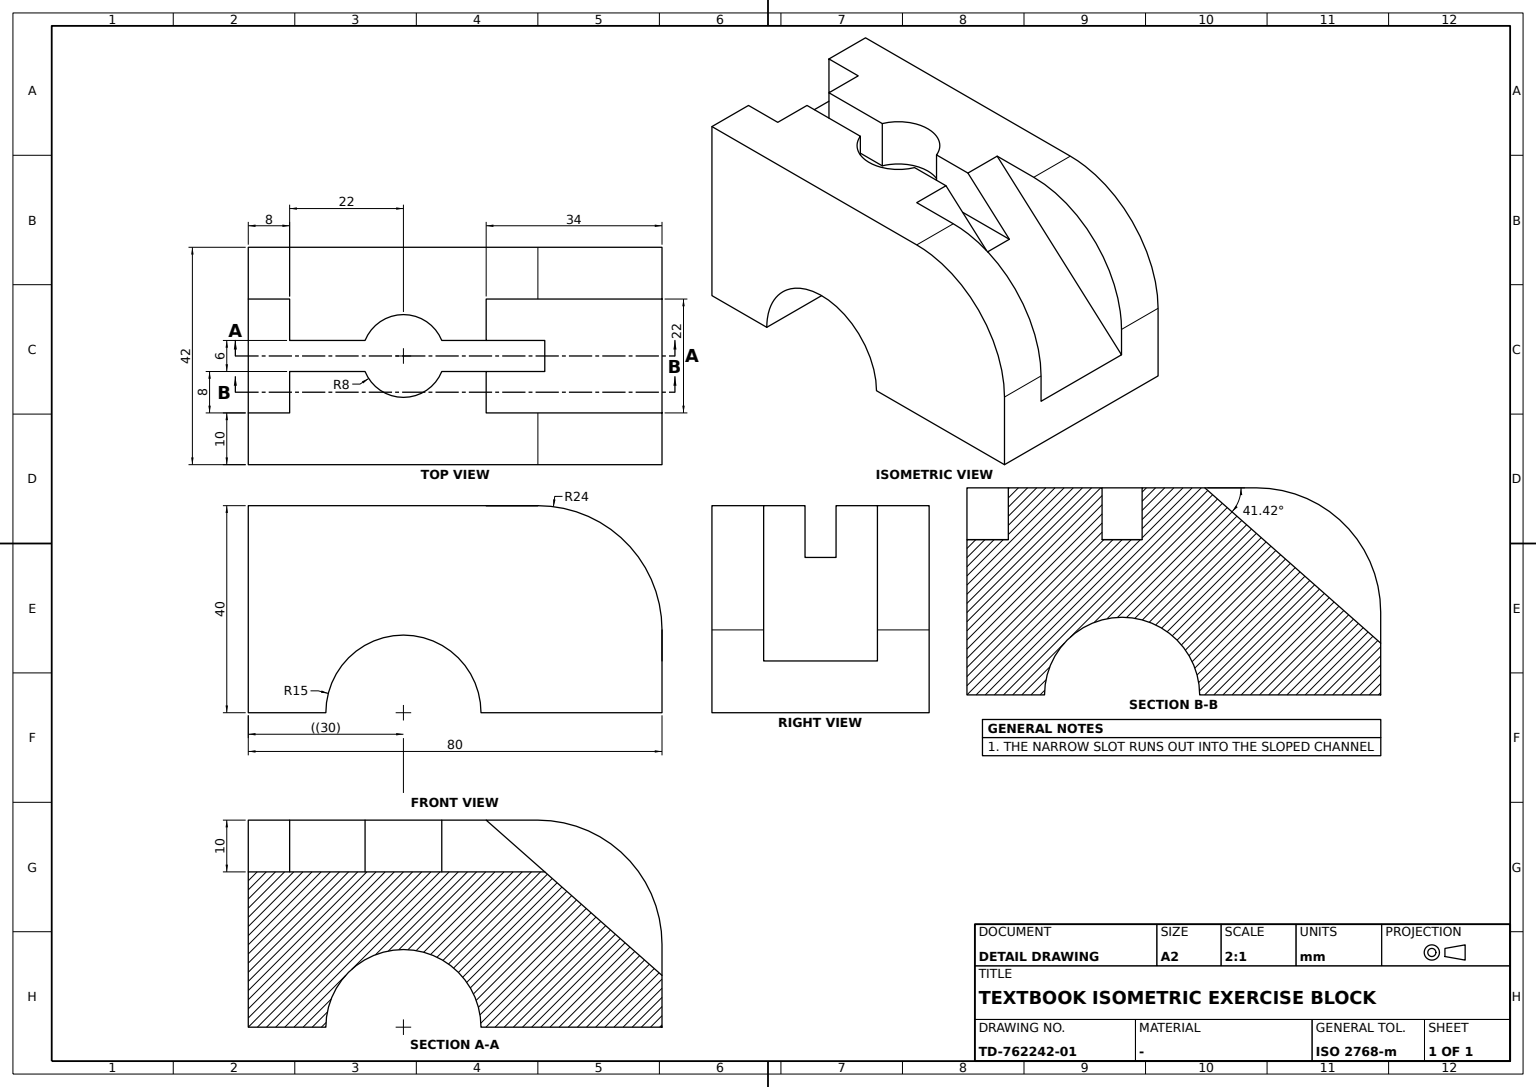
ISO-10303-21;
HEADER;
FILE_DESCRIPTION((''),'2;1');
FILE_NAME('','',(''),(''),'','','');
FILE_SCHEMA(('AUTOMOTIVE_DESIGN'));
ENDSEC;
DATA;
#1=APPLICATION_CONTEXT('');
#2=PRODUCT_CONTEXT('',#1,'mechanical');
#3=PRODUCT('','','',(#2));
#4=PRODUCT_DEFINITION_FORMATION('','',#3);
#5=PRODUCT_DEFINITION_CONTEXT('',#1,'design');
#6=PRODUCT_DEFINITION('','',#4,#5);
#7=PRODUCT_DEFINITION_SHAPE('','',#6);
#8=(LENGTH_UNIT()NAMED_UNIT(*)SI_UNIT(.MILLI.,.METRE.));
#9=(NAMED_UNIT(*)PLANE_ANGLE_UNIT()SI_UNIT($,.RADIAN.));
#10=(NAMED_UNIT(*)SI_UNIT($,.STERADIAN.)SOLID_ANGLE_UNIT());
#11=UNCERTAINTY_MEASURE_WITH_UNIT(LENGTH_MEASURE(0.005),#8,'distance_accuracy_value','');
#12=(GEOMETRIC_REPRESENTATION_CONTEXT(3)GLOBAL_UNCERTAINTY_ASSIGNED_CONTEXT((#11))GLOBAL_UNIT_ASSIGNED_CONTEXT((#8,#9,#10))REPRESENTATION_CONTEXT('',''));
#13=CARTESIAN_POINT('',(21.,0.,0.));
#14=VERTEX_POINT('',#13);
#15=CARTESIAN_POINT('',(21.,15.,0.));
#16=VERTEX_POINT('',#15);
#17=DIRECTION('',(0.,1.,0.));
#18=VECTOR('',#17,1000.);
#19=LINE('',#13,#18);
#20=EDGE_CURVE('',#14,#16,#19,.T.);
#21=ORIENTED_EDGE('',*,*,#20,.T.);
#22=CARTESIAN_POINT('',(21.,45.,0.));
#23=VERTEX_POINT('',#22);
#24=CARTESIAN_POINT('',(21.,30.,0.));
#25=DIRECTION('',(1.,0.,0.));
#26=DIRECTION('',(0.,0.,-1.));
#27=AXIS2_PLACEMENT_3D('',#24,#25,#26);
#28=CIRCLE('',#27,15.);
#29=EDGE_CURVE('',#23,#16,#28,.T.);
#30=ORIENTED_EDGE('',*,*,#29,.F.);
#31=CARTESIAN_POINT('',(21.,80.,0.));
#32=VERTEX_POINT('',#31);
#33=EDGE_CURVE('',#23,#32,#19,.T.);
#34=ORIENTED_EDGE('',*,*,#33,.T.);
#35=CARTESIAN_POINT('',(21.,80.,16.));
#36=VERTEX_POINT('',#35);
#37=DIRECTION('',(0.,0.,1.));
#38=VECTOR('',#37,1000.);
#39=LINE('',#31,#38);
#40=EDGE_CURVE('',#32,#36,#39,.T.);
#41=ORIENTED_EDGE('',*,*,#40,.T.);
#42=CARTESIAN_POINT('',(21.,56.,40.));
#43=VERTEX_POINT('',#42);
#44=CARTESIAN_POINT('',(21.,56.,16.));
#45=AXIS2_PLACEMENT_3D('',#44,#25,#26);
#46=CIRCLE('',#45,24.);
#47=EDGE_CURVE('',#36,#43,#46,.T.);
#48=ORIENTED_EDGE('',*,*,#47,.T.);
#49=CARTESIAN_POINT('',(21.,0.,40.));
#50=VERTEX_POINT('',#49);
#51=DIRECTION('',(0.,-1.,0.));
#52=VECTOR('',#51,1000.);
#53=LINE('',#49,#52);
#54=EDGE_CURVE('',#43,#50,#53,.T.);
#55=ORIENTED_EDGE('',*,*,#54,.T.);
#56=VECTOR('',#26,1000.);
#57=LINE('',#13,#56);
#58=EDGE_CURVE('',#50,#14,#57,.T.);
#59=ORIENTED_EDGE('',*,*,#58,.T.);
#60=EDGE_LOOP('',(#21,#30,#34,#41,#48,#55,#59));
#61=FACE_BOUND('',#60,.T.);
#62=AXIS2_PLACEMENT_3D('',#13,#25,#17);
#63=PLANE('',#62);
#64=ADVANCED_FACE('',(#61),#63,.T.);
#65=CARTESIAN_POINT('',(3.,22.583802,40.));
#66=VERTEX_POINT('',#65);
#67=CARTESIAN_POINT('',(3.,37.416198,40.));
#68=VERTEX_POINT('',#67);
#69=CARTESIAN_POINT('',(0.,30.,40.));
#70=AXIS2_PLACEMENT_3D('',#69,#37,#25);
#71=CIRCLE('',#70,8.);
#72=EDGE_CURVE('',#66,#68,#71,.T.);
#73=ORIENTED_EDGE('',*,*,#72,.T.);
#74=CARTESIAN_POINT('',(3.,37.416198,30.));
#75=VERTEX_POINT('',#74);
#76=LINE('',#67,#38);
#77=EDGE_CURVE('',#68,#75,#76,.F.);
#78=ORIENTED_EDGE('',*,*,#77,.T.);
#79=CARTESIAN_POINT('',(3.,22.583802,30.));
#80=VERTEX_POINT('',#79);
#81=CARTESIAN_POINT('',(0.,30.,30.));
#82=AXIS2_PLACEMENT_3D('',#81,#37,#25);
#83=CIRCLE('',#82,8.);
#84=EDGE_CURVE('',#80,#75,#83,.T.);
#85=ORIENTED_EDGE('',*,*,#84,.F.);
#86=LINE('',#65,#38);
#87=EDGE_CURVE('',#66,#80,#86,.F.);
#88=ORIENTED_EDGE('',*,*,#87,.F.);
#89=EDGE_LOOP('',(#73,#78,#85,#88));
#90=FACE_BOUND('',#89,.T.);
#91=CARTESIAN_POINT('',(0.,30.,35.));
#92=AXIS2_PLACEMENT_3D('',#91,#37,#25);
#93=CYLINDRICAL_SURFACE('',#92,8.);
#94=ADVANCED_FACE('',(#90),#93,.F.);
#95=CARTESIAN_POINT('',(-11.,56.,40.));
#96=VERTEX_POINT('',#95);
#97=CARTESIAN_POINT('',(-11.,80.,16.));
#98=VERTEX_POINT('',#97);
#99=CARTESIAN_POINT('',(-11.,56.,16.));
#100=DIRECTION('',(-1.,0.,0.));
#101=AXIS2_PLACEMENT_3D('',#99,#100,#37);
#102=CIRCLE('',#101,24.);
#103=EDGE_CURVE('',#96,#98,#102,.T.);
#104=ORIENTED_EDGE('',*,*,#103,.T.);
#105=CARTESIAN_POINT('',(-21.,80.,16.));
#106=VERTEX_POINT('',#105);
#107=CARTESIAN_POINT('',(0.,80.,16.));
#108=VECTOR('',#25,1000.);
#109=LINE('',#107,#108);
#110=EDGE_CURVE('',#106,#98,#109,.T.);
#111=ORIENTED_EDGE('',*,*,#110,.F.);
#112=CARTESIAN_POINT('',(-21.,56.,40.));
#113=VERTEX_POINT('',#112);
#114=CARTESIAN_POINT('',(-21.,56.,16.));
#115=AXIS2_PLACEMENT_3D('',#114,#25,#26);
#116=CIRCLE('',#115,24.);
#117=EDGE_CURVE('',#106,#113,#116,.T.);
#118=ORIENTED_EDGE('',*,*,#117,.T.);
#119=CARTESIAN_POINT('',(0.,56.,40.));
#120=LINE('',#119,#108);
#121=EDGE_CURVE('',#113,#96,#120,.T.);
#122=ORIENTED_EDGE('',*,*,#121,.T.);
#123=EDGE_LOOP('',(#104,#111,#118,#122));
#124=FACE_BOUND('',#123,.T.);
#125=CARTESIAN_POINT('',(0.,56.,16.));
#126=AXIS2_PLACEMENT_3D('',#125,#25,#37);
#127=CYLINDRICAL_SURFACE('',#126,24.);
#128=ADVANCED_FACE('',(#124),#127,.T.);
#129=CARTESIAN_POINT('',(-3.,46.,40.));
#130=VERTEX_POINT('',#129);
#131=CARTESIAN_POINT('',(-3.,57.333333,30.));
#132=VERTEX_POINT('',#131);
#133=DIRECTION('',(0.,0.749837855,-0.661621637));
#134=VECTOR('',#133,1000.);
#135=LINE('',#129,#134);
#136=EDGE_CURVE('',#130,#132,#135,.T.);
#137=ORIENTED_EDGE('',*,*,#136,.F.);
#138=CARTESIAN_POINT('',(-3.,37.416198,40.));
#139=VERTEX_POINT('',#138);
#140=CARTESIAN_POINT('',(-3.,57.416198,40.));
#141=LINE('',#140,#52);
#142=EDGE_CURVE('',#130,#139,#141,.T.);
#143=ORIENTED_EDGE('',*,*,#142,.T.);
#144=CARTESIAN_POINT('',(-3.,37.416198,30.));
#145=VERTEX_POINT('',#144);
#146=LINE('',#138,#38);
#147=EDGE_CURVE('',#139,#145,#146,.F.);
#148=ORIENTED_EDGE('',*,*,#147,.T.);
#149=CARTESIAN_POINT('',(-3.,57.416198,30.));
#150=LINE('',#149,#52);
#151=EDGE_CURVE('',#132,#145,#150,.T.);
#152=ORIENTED_EDGE('',*,*,#151,.F.);
#153=EDGE_LOOP('',(#137,#143,#148,#152));
#154=FACE_BOUND('',#153,.T.);
#155=AXIS2_PLACEMENT_3D('',#140,#25,#51);
#156=PLANE('',#155);
#157=ADVANCED_FACE('',(#154),#156,.T.);
#158=ORIENTED_EDGE('',*,*,#84,.T.);
#159=CARTESIAN_POINT('',(3.,57.333333,30.));
#160=VERTEX_POINT('',#159);
#161=CARTESIAN_POINT('',(3.,8.,30.));
#162=LINE('',#161,#18);
#163=EDGE_CURVE('',#75,#160,#162,.T.);
#164=ORIENTED_EDGE('',*,*,#163,.T.);
#165=CARTESIAN_POINT('',(21.,57.333333,30.));
#166=LINE('',#165,#108);
#167=EDGE_CURVE('',#132,#160,#166,.T.);
#168=ORIENTED_EDGE('',*,*,#167,.F.);
#169=ORIENTED_EDGE('',*,*,#151,.T.);
#170=CARTESIAN_POINT('',(-3.,22.583802,30.));
#171=VERTEX_POINT('',#170);
#172=EDGE_CURVE('',#145,#171,#83,.T.);
#173=ORIENTED_EDGE('',*,*,#172,.T.);
#174=CARTESIAN_POINT('',(-3.,8.,30.));
#175=VERTEX_POINT('',#174);
#176=EDGE_CURVE('',#171,#175,#150,.T.);
#177=ORIENTED_EDGE('',*,*,#176,.T.);
#178=CARTESIAN_POINT('',(-11.,8.,30.));
#179=VERTEX_POINT('',#178);
#180=LINE('',#161,#108);
#181=EDGE_CURVE('',#179,#175,#180,.T.);
#182=ORIENTED_EDGE('',*,*,#181,.F.);
#183=CARTESIAN_POINT('',(-11.,0.,30.));
#184=VERTEX_POINT('',#183);
#185=LINE('',#183,#52);
#186=EDGE_CURVE('',#179,#184,#185,.T.);
#187=ORIENTED_EDGE('',*,*,#186,.T.);
#188=CARTESIAN_POINT('',(11.,0.,30.));
#189=VERTEX_POINT('',#188);
#190=CARTESIAN_POINT('',(0.,0.,30.));
#191=VECTOR('',#100,1000.);
#192=LINE('',#190,#191);
#193=EDGE_CURVE('',#189,#184,#192,.T.);
#194=ORIENTED_EDGE('',*,*,#193,.F.);
#195=CARTESIAN_POINT('',(11.,8.,30.));
#196=VERTEX_POINT('',#195);
#197=LINE('',#188,#18);
#198=EDGE_CURVE('',#189,#196,#197,.T.);
#199=ORIENTED_EDGE('',*,*,#198,.T.);
#200=VERTEX_POINT('',#161);
#201=EDGE_CURVE('',#200,#196,#180,.T.);
#202=ORIENTED_EDGE('',*,*,#201,.F.);
#203=EDGE_CURVE('',#200,#80,#162,.T.);
#204=ORIENTED_EDGE('',*,*,#203,.T.);
#205=EDGE_LOOP('',(#158,#164,#168,#169,#173,#177,#182,#187,#194,#199,#202,#204));
#206=FACE_BOUND('',#205,.T.);
#207=AXIS2_PLACEMENT_3D('',#190,#37,#25);
#208=PLANE('',#207);
#209=ADVANCED_FACE('',(#206),#208,.T.);
#210=ORIENTED_EDGE('',*,*,#186,.F.);
#211=CARTESIAN_POINT('',(-11.,8.,40.));
#212=VERTEX_POINT('',#211);
#213=CARTESIAN_POINT('',(-11.,8.,0.));
#214=LINE('',#213,#56);
#215=EDGE_CURVE('',#212,#179,#214,.T.);
#216=ORIENTED_EDGE('',*,*,#215,.F.);
#217=CARTESIAN_POINT('',(-11.,0.,40.));
#218=VERTEX_POINT('',#217);
#219=CARTESIAN_POINT('',(-11.,80.,40.));
#220=LINE('',#219,#52);
#221=EDGE_CURVE('',#212,#218,#220,.T.);
#222=ORIENTED_EDGE('',*,*,#221,.T.);
#223=LINE('',#217,#56);
#224=EDGE_CURVE('',#218,#184,#223,.T.);
#225=ORIENTED_EDGE('',*,*,#224,.T.);
#226=EDGE_LOOP('',(#210,#216,#222,#225));
#227=FACE_BOUND('',#226,.T.);
#228=CARTESIAN_POINT('',(-11.,0.,0.));
#229=AXIS2_PLACEMENT_3D('',#228,#100,#51);
#230=PLANE('',#229);
#231=ADVANCED_FACE('',(#227),#230,.F.);
#232=CARTESIAN_POINT('',(-21.,0.,0.));
#233=VERTEX_POINT('',#232);
#234=CARTESIAN_POINT('',(0.,0.,0.));
#235=LINE('',#234,#108);
#236=EDGE_CURVE('',#233,#14,#235,.T.);
#237=ORIENTED_EDGE('',*,*,#236,.F.);
#238=CARTESIAN_POINT('',(-21.,15.,0.));
#239=VERTEX_POINT('',#238);
#240=LINE('',#232,#18);
#241=EDGE_CURVE('',#233,#239,#240,.T.);
#242=ORIENTED_EDGE('',*,*,#241,.T.);
#243=LINE('',#238,#108);
#244=EDGE_CURVE('',#239,#16,#243,.T.);
#245=ORIENTED_EDGE('',*,*,#244,.T.);
#246=ORIENTED_EDGE('',*,*,#20,.F.);
#247=EDGE_LOOP('',(#237,#242,#245,#246));
#248=FACE_BOUND('',#247,.T.);
#249=AXIS2_PLACEMENT_3D('',#234,#26,#17);
#250=PLANE('',#249);
#251=ADVANCED_FACE('',(#248),#250,.T.);
#252=ORIENTED_EDGE('',*,*,#201,.T.);
#253=CARTESIAN_POINT('',(11.,8.,40.));
#254=VERTEX_POINT('',#253);
#255=LINE('',#253,#56);
#256=EDGE_CURVE('',#254,#196,#255,.T.);
#257=ORIENTED_EDGE('',*,*,#256,.F.);
#258=CARTESIAN_POINT('',(3.,8.,40.));
#259=VERTEX_POINT('',#258);
#260=LINE('',#258,#108);
#261=EDGE_CURVE('',#259,#254,#260,.T.);
#262=ORIENTED_EDGE('',*,*,#261,.F.);
#263=LINE('',#258,#56);
#264=EDGE_CURVE('',#259,#200,#263,.T.);
#265=ORIENTED_EDGE('',*,*,#264,.T.);
#266=EDGE_LOOP('',(#252,#257,#262,#265));
#267=FACE_BOUND('',#266,.T.);
#268=AXIS2_PLACEMENT_3D('',#258,#17,#25);
#269=PLANE('',#268);
#270=ADVANCED_FACE('',(#267),#269,.F.);
#271=CARTESIAN_POINT('',(11.,80.,16.));
#272=VERTEX_POINT('',#271);
#273=EDGE_CURVE('',#36,#272,#109,.F.);
#274=ORIENTED_EDGE('',*,*,#273,.F.);
#275=ORIENTED_EDGE('',*,*,#40,.F.);
#276=CARTESIAN_POINT('',(-21.,80.,0.));
#277=VERTEX_POINT('',#276);
#278=CARTESIAN_POINT('',(0.,80.,0.));
#279=LINE('',#278,#108);
#280=EDGE_CURVE('',#277,#32,#279,.T.);
#281=ORIENTED_EDGE('',*,*,#280,.F.);
#282=LINE('',#276,#38);
#283=EDGE_CURVE('',#277,#106,#282,.T.);
#284=ORIENTED_EDGE('',*,*,#283,.T.);
#285=ORIENTED_EDGE('',*,*,#110,.T.);
#286=CARTESIAN_POINT('',(-11.,80.,10.));
#287=VERTEX_POINT('',#286);
#288=CARTESIAN_POINT('',(-11.,80.,0.));
#289=LINE('',#288,#38);
#290=EDGE_CURVE('',#287,#98,#289,.T.);
#291=ORIENTED_EDGE('',*,*,#290,.F.);
#292=CARTESIAN_POINT('',(11.,80.,10.));
#293=VERTEX_POINT('',#292);
#294=CARTESIAN_POINT('',(21.,80.,10.));
#295=LINE('',#294,#191);
#296=EDGE_CURVE('',#293,#287,#295,.T.);
#297=ORIENTED_EDGE('',*,*,#296,.F.);
#298=CARTESIAN_POINT('',(11.,80.,0.));
#299=LINE('',#298,#38);
#300=EDGE_CURVE('',#293,#272,#299,.T.);
#301=ORIENTED_EDGE('',*,*,#300,.T.);
#302=EDGE_LOOP('',(#274,#275,#281,#284,#285,#291,#297,#301));
#303=FACE_BOUND('',#302,.T.);
#304=AXIS2_PLACEMENT_3D('',#278,#17,#37);
#305=PLANE('',#304);
#306=ADVANCED_FACE('',(#303),#305,.T.);
#307=CARTESIAN_POINT('',(-21.,0.,40.));
#308=VERTEX_POINT('',#307);
#309=LINE('',#232,#56);
#310=EDGE_CURVE('',#308,#233,#309,.T.);
#311=ORIENTED_EDGE('',*,*,#310,.T.);
#312=ORIENTED_EDGE('',*,*,#236,.T.);
#313=ORIENTED_EDGE('',*,*,#58,.F.);
#314=CARTESIAN_POINT('',(11.,0.,40.));
#315=VERTEX_POINT('',#314);
#316=CARTESIAN_POINT('',(0.,0.,40.));
#317=LINE('',#316,#108);
#318=EDGE_CURVE('',#315,#50,#317,.T.);
#319=ORIENTED_EDGE('',*,*,#318,.F.);
#320=CARTESIAN_POINT('',(11.,0.,0.));
#321=LINE('',#320,#56);
#322=EDGE_CURVE('',#315,#189,#321,.T.);
#323=ORIENTED_EDGE('',*,*,#322,.T.);
#324=ORIENTED_EDGE('',*,*,#193,.T.);
#325=ORIENTED_EDGE('',*,*,#224,.F.);
#326=EDGE_CURVE('',#308,#218,#317,.T.);
#327=ORIENTED_EDGE('',*,*,#326,.F.);
#328=EDGE_LOOP('',(#311,#312,#313,#319,#323,#324,#325,#327));
#329=FACE_BOUND('',#328,.T.);
#330=AXIS2_PLACEMENT_3D('',#316,#51,#26);
#331=PLANE('',#330);
#332=ADVANCED_FACE('',(#329),#331,.T.);
#333=ORIENTED_EDGE('',*,*,#87,.T.);
#334=ORIENTED_EDGE('',*,*,#203,.F.);
#335=ORIENTED_EDGE('',*,*,#264,.F.);
#336=LINE('',#258,#18);
#337=EDGE_CURVE('',#259,#66,#336,.T.);
#338=ORIENTED_EDGE('',*,*,#337,.T.);
#339=EDGE_LOOP('',(#333,#334,#335,#338));
#340=FACE_BOUND('',#339,.T.);
#341=AXIS2_PLACEMENT_3D('',#258,#100,#17);
#342=PLANE('',#341);
#343=ADVANCED_FACE('',(#340),#342,.T.);
#344=CARTESIAN_POINT('',(11.,46.,40.));
#345=VERTEX_POINT('',#344);
#346=LINE('',#344,#134);
#347=EDGE_CURVE('',#345,#293,#346,.T.);
#348=ORIENTED_EDGE('',*,*,#347,.F.);
#349=CARTESIAN_POINT('',(11.,56.,40.));
#350=VERTEX_POINT('',#349);
#351=LINE('',#314,#52);
#352=EDGE_CURVE('',#350,#345,#351,.T.);
#353=ORIENTED_EDGE('',*,*,#352,.F.);
#354=CARTESIAN_POINT('',(11.,56.,16.));
#355=AXIS2_PLACEMENT_3D('',#354,#25,#26);
#356=CIRCLE('',#355,24.);
#357=EDGE_CURVE('',#272,#350,#356,.T.);
#358=ORIENTED_EDGE('',*,*,#357,.F.);
#359=ORIENTED_EDGE('',*,*,#300,.F.);
#360=EDGE_LOOP('',(#348,#353,#358,#359));
#361=FACE_BOUND('',#360,.T.);
#362=AXIS2_PLACEMENT_3D('',#320,#25,#17);
#363=PLANE('',#362);
#364=ADVANCED_FACE('',(#361),#363,.F.);
#365=ORIENTED_EDGE('',*,*,#326,.T.);
#366=ORIENTED_EDGE('',*,*,#221,.F.);
#367=CARTESIAN_POINT('',(-3.,8.,40.));
#368=VERTEX_POINT('',#367);
#369=EDGE_CURVE('',#212,#368,#260,.T.);
#370=ORIENTED_EDGE('',*,*,#369,.T.);
#371=CARTESIAN_POINT('',(-3.,22.583802,40.));
#372=VERTEX_POINT('',#371);
#373=EDGE_CURVE('',#372,#368,#141,.T.);
#374=ORIENTED_EDGE('',*,*,#373,.F.);
#375=EDGE_CURVE('',#139,#372,#71,.T.);
#376=ORIENTED_EDGE('',*,*,#375,.F.);
#377=ORIENTED_EDGE('',*,*,#142,.F.);
#378=CARTESIAN_POINT('',(-11.,46.,40.));
#379=VERTEX_POINT('',#378);
#380=CARTESIAN_POINT('',(0.,46.,40.));
#381=LINE('',#380,#191);
#382=EDGE_CURVE('',#130,#379,#381,.T.);
#383=ORIENTED_EDGE('',*,*,#382,.T.);
#384=EDGE_CURVE('',#96,#379,#220,.T.);
#385=ORIENTED_EDGE('',*,*,#384,.F.);
#386=ORIENTED_EDGE('',*,*,#121,.F.);
#387=LINE('',#307,#52);
#388=EDGE_CURVE('',#113,#308,#387,.T.);
#389=ORIENTED_EDGE('',*,*,#388,.T.);
#390=EDGE_LOOP('',(#365,#366,#370,#374,#376,#377,#383,#385,#386,#389));
#391=FACE_BOUND('',#390,.T.);
#392=CARTESIAN_POINT('',(0.,80.,40.));
#393=AXIS2_PLACEMENT_3D('',#392,#37,#51);
#394=PLANE('',#393);
#395=ADVANCED_FACE('',(#391),#394,.T.);
#396=ORIENTED_EDGE('',*,*,#33,.F.);
#397=CARTESIAN_POINT('',(-21.,45.,0.));
#398=VERTEX_POINT('',#397);
#399=LINE('',#397,#108);
#400=EDGE_CURVE('',#23,#398,#399,.F.);
#401=ORIENTED_EDGE('',*,*,#400,.T.);
#402=EDGE_CURVE('',#398,#277,#240,.T.);
#403=ORIENTED_EDGE('',*,*,#402,.T.);
#404=ORIENTED_EDGE('',*,*,#280,.T.);
#405=EDGE_LOOP('',(#396,#401,#403,#404));
#406=FACE_BOUND('',#405,.T.);
#407=ADVANCED_FACE('',(#406),#250,.T.);
#408=LINE('',#371,#38);
#409=EDGE_CURVE('',#372,#171,#408,.F.);
#410=ORIENTED_EDGE('',*,*,#409,.F.);
#411=ORIENTED_EDGE('',*,*,#373,.T.);
#412=LINE('',#367,#56);
#413=EDGE_CURVE('',#368,#175,#412,.T.);
#414=ORIENTED_EDGE('',*,*,#413,.T.);
#415=ORIENTED_EDGE('',*,*,#176,.F.);
#416=EDGE_LOOP('',(#410,#411,#414,#415));
#417=FACE_BOUND('',#416,.T.);
#418=ADVANCED_FACE('',(#417),#156,.T.);
#419=ORIENTED_EDGE('',*,*,#413,.F.);
#420=ORIENTED_EDGE('',*,*,#369,.F.);
#421=ORIENTED_EDGE('',*,*,#215,.T.);
#422=ORIENTED_EDGE('',*,*,#181,.T.);
#423=EDGE_LOOP('',(#419,#420,#421,#422));
#424=FACE_BOUND('',#423,.T.);
#425=ADVANCED_FACE('',(#424),#269,.F.);
#426=ORIENTED_EDGE('',*,*,#375,.T.);
#427=ORIENTED_EDGE('',*,*,#409,.T.);
#428=ORIENTED_EDGE('',*,*,#172,.F.);
#429=ORIENTED_EDGE('',*,*,#147,.F.);
#430=EDGE_LOOP('',(#426,#427,#428,#429));
#431=FACE_BOUND('',#430,.T.);
#432=ADVANCED_FACE('',(#431),#93,.F.);
#433=ORIENTED_EDGE('',*,*,#163,.F.);
#434=ORIENTED_EDGE('',*,*,#77,.F.);
#435=CARTESIAN_POINT('',(3.,46.,40.));
#436=VERTEX_POINT('',#435);
#437=EDGE_CURVE('',#68,#436,#336,.T.);
#438=ORIENTED_EDGE('',*,*,#437,.T.);
#439=CARTESIAN_POINT('',(3.,24.634241,58.85214));
#440=LINE('',#439,#134);
#441=EDGE_CURVE('',#436,#160,#440,.T.);
#442=ORIENTED_EDGE('',*,*,#441,.T.);
#443=EDGE_LOOP('',(#433,#434,#438,#442));
#444=FACE_BOUND('',#443,.T.);
#445=ADVANCED_FACE('',(#444),#342,.T.);
#446=EDGE_CURVE('',#345,#436,#381,.T.);
#447=ORIENTED_EDGE('',*,*,#446,.T.);
#448=ORIENTED_EDGE('',*,*,#437,.F.);
#449=ORIENTED_EDGE('',*,*,#72,.F.);
#450=ORIENTED_EDGE('',*,*,#337,.F.);
#451=ORIENTED_EDGE('',*,*,#261,.T.);
#452=CARTESIAN_POINT('',(11.,80.,40.));
#453=LINE('',#452,#18);
#454=EDGE_CURVE('',#315,#254,#453,.T.);
#455=ORIENTED_EDGE('',*,*,#454,.F.);
#456=ORIENTED_EDGE('',*,*,#318,.T.);
#457=ORIENTED_EDGE('',*,*,#54,.F.);
#458=EDGE_CURVE('',#43,#350,#120,.F.);
#459=ORIENTED_EDGE('',*,*,#458,.T.);
#460=ORIENTED_EDGE('',*,*,#352,.T.);
#461=EDGE_LOOP('',(#447,#448,#449,#450,#451,#455,#456,#457,#459,#460));
#462=FACE_BOUND('',#461,.T.);
#463=ADVANCED_FACE('',(#462),#394,.T.);
#464=ORIENTED_EDGE('',*,*,#388,.F.);
#465=ORIENTED_EDGE('',*,*,#117,.F.);
#466=ORIENTED_EDGE('',*,*,#283,.F.);
#467=ORIENTED_EDGE('',*,*,#402,.F.);
#468=CARTESIAN_POINT('',(-21.,30.,0.));
#469=AXIS2_PLACEMENT_3D('',#468,#25,#26);
#470=CIRCLE('',#469,15.);
#471=EDGE_CURVE('',#398,#239,#470,.T.);
#472=ORIENTED_EDGE('',*,*,#471,.T.);
#473=ORIENTED_EDGE('',*,*,#241,.F.);
#474=ORIENTED_EDGE('',*,*,#310,.F.);
#475=EDGE_LOOP('',(#464,#465,#466,#467,#472,#473,#474));
#476=FACE_BOUND('',#475,.T.);
#477=AXIS2_PLACEMENT_3D('',#232,#25,#17);
#478=PLANE('',#477);
#479=ADVANCED_FACE('',(#476),#478,.F.);
#480=ORIENTED_EDGE('',*,*,#47,.F.);
#481=ORIENTED_EDGE('',*,*,#273,.T.);
#482=ORIENTED_EDGE('',*,*,#357,.T.);
#483=ORIENTED_EDGE('',*,*,#458,.F.);
#484=EDGE_LOOP('',(#480,#481,#482,#483));
#485=FACE_BOUND('',#484,.T.);
#486=ADVANCED_FACE('',(#485),#127,.T.);
#487=CARTESIAN_POINT('',(-11.,39.980545,45.311284));
#488=LINE('',#487,#134);
#489=EDGE_CURVE('',#379,#287,#488,.T.);
#490=ORIENTED_EDGE('',*,*,#489,.T.);
#491=ORIENTED_EDGE('',*,*,#290,.T.);
#492=ORIENTED_EDGE('',*,*,#103,.F.);
#493=ORIENTED_EDGE('',*,*,#384,.T.);
#494=EDGE_LOOP('',(#490,#491,#492,#493));
#495=FACE_BOUND('',#494,.T.);
#496=ADVANCED_FACE('',(#495),#230,.F.);
#497=ORIENTED_EDGE('',*,*,#136,.T.);
#498=ORIENTED_EDGE('',*,*,#167,.T.);
#499=ORIENTED_EDGE('',*,*,#441,.F.);
#500=ORIENTED_EDGE('',*,*,#446,.F.);
#501=ORIENTED_EDGE('',*,*,#347,.T.);
#502=ORIENTED_EDGE('',*,*,#296,.T.);
#503=ORIENTED_EDGE('',*,*,#489,.F.);
#504=ORIENTED_EDGE('',*,*,#382,.F.);
#505=EDGE_LOOP('',(#497,#498,#499,#500,#501,#502,#503,#504));
#506=FACE_BOUND('',#505,.T.);
#507=CARTESIAN_POINT('',(21.,46.,40.));
#508=DIRECTION('',(0.,0.661621637,0.749837855));
#509=AXIS2_PLACEMENT_3D('',#507,#508,#133);
#510=PLANE('',#509);
#511=ADVANCED_FACE('',(#506),#510,.T.);
#512=ORIENTED_EDGE('',*,*,#322,.F.);
#513=ORIENTED_EDGE('',*,*,#454,.T.);
#514=ORIENTED_EDGE('',*,*,#256,.T.);
#515=ORIENTED_EDGE('',*,*,#198,.F.);
#516=EDGE_LOOP('',(#512,#513,#514,#515));
#517=FACE_BOUND('',#516,.T.);
#518=ADVANCED_FACE('',(#517),#363,.F.);
#519=ORIENTED_EDGE('',*,*,#29,.T.);
#520=ORIENTED_EDGE('',*,*,#244,.F.);
#521=ORIENTED_EDGE('',*,*,#471,.F.);
#522=ORIENTED_EDGE('',*,*,#400,.F.);
#523=EDGE_LOOP('',(#519,#520,#521,#522));
#524=FACE_BOUND('',#523,.T.);
#525=CARTESIAN_POINT('',(-0.66,30.,0.));
#526=AXIS2_PLACEMENT_3D('',#525,#25,#17);
#527=CYLINDRICAL_SURFACE('',#526,15.);
#528=ADVANCED_FACE('',(#524),#527,.F.);
#529=CLOSED_SHELL('',(#64,#94,#128,#157,#209,#231,#251,#270,#306,#332,#343,#364,#395,#407,#418,#425,#432,#445,#463,#479,#486,#496,#511,#518,#528));
#530=MANIFOLD_SOLID_BREP('',#529);
#531=ADVANCED_BREP_SHAPE_REPRESENTATION('',(#530),#12);
#532=SHAPE_DEFINITION_REPRESENTATION(#7,#531);
ENDSEC;
END-ISO-10303-21;
